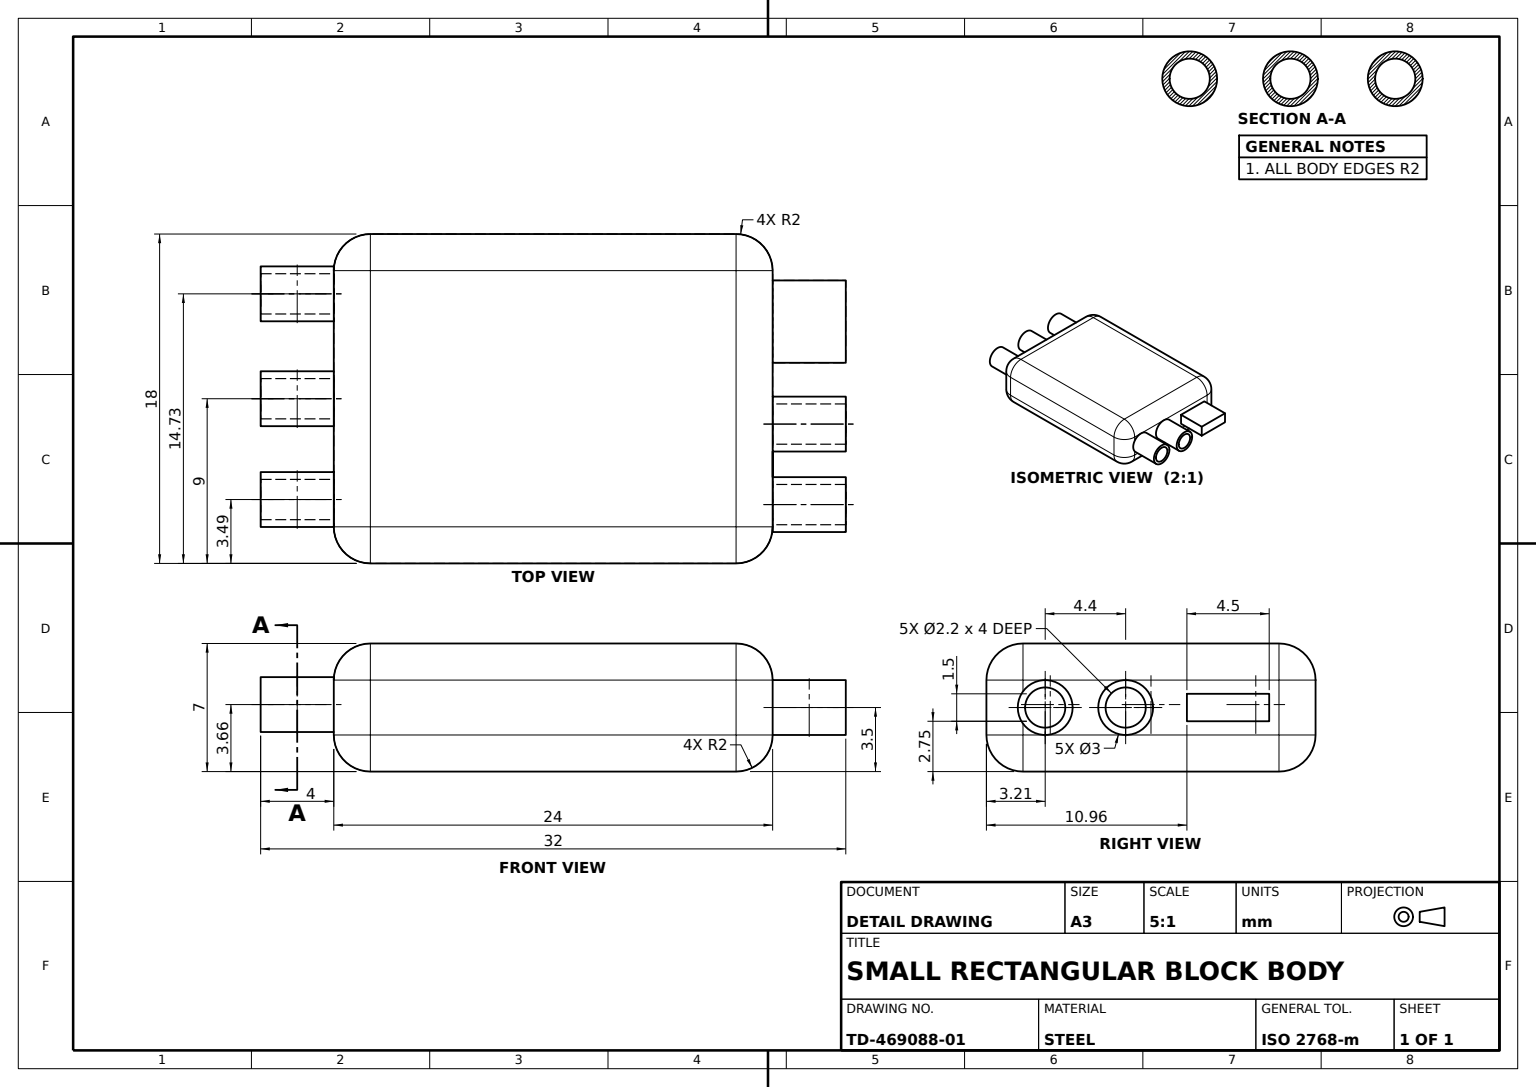
ISO-10303-21;
HEADER;
FILE_DESCRIPTION((''),'2;1');
FILE_NAME('','',(''),(''),'','','');
FILE_SCHEMA(('AUTOMOTIVE_DESIGN'));
ENDSEC;
DATA;
#1=APPLICATION_CONTEXT('');
#2=PRODUCT_CONTEXT('',#1,'mechanical');
#3=PRODUCT('','','',(#2));
#4=PRODUCT_DEFINITION_FORMATION('','',#3);
#5=PRODUCT_DEFINITION_CONTEXT('',#1,'design');
#6=PRODUCT_DEFINITION('','',#4,#5);
#7=PRODUCT_DEFINITION_SHAPE('','',#6);
#8=(LENGTH_UNIT()NAMED_UNIT(*)SI_UNIT(.MILLI.,.METRE.));
#9=(NAMED_UNIT(*)PLANE_ANGLE_UNIT()SI_UNIT($,.RADIAN.));
#10=(NAMED_UNIT(*)SI_UNIT($,.STERADIAN.)SOLID_ANGLE_UNIT());
#11=UNCERTAINTY_MEASURE_WITH_UNIT(LENGTH_MEASURE(1.E-05),#8,'distance_accuracy_value','');
#12=(GEOMETRIC_REPRESENTATION_CONTEXT(3)GLOBAL_UNCERTAINTY_ASSIGNED_CONTEXT((#11))GLOBAL_UNIT_ASSIGNED_CONTEXT((#8,#9,#10))REPRESENTATION_CONTEXT('',''));
#13=CARTESIAN_POINT('',(12.,2.,7.));
#14=VERTEX_POINT('',#13);
#15=CARTESIAN_POINT('',(12.,2.,5.785269));
#16=VERTEX_POINT('',#15);
#17=CARTESIAN_POINT('',(12.,2.,-7.));
#18=DIRECTION('',(0.,0.,-1.));
#19=VECTOR('',#18,1000.);
#20=LINE('',#17,#19);
#21=EDGE_CURVE('',#14,#16,#20,.T.);
#22=ORIENTED_EDGE('',*,*,#21,.T.);
#23=CARTESIAN_POINT('',(12.,2.619984,7.));
#24=VERTEX_POINT('',#23);
#25=CARTESIAN_POINT('',(12.,3.5,5.785269));
#26=DIRECTION('',(1.,0.,0.));
#27=AXIS2_PLACEMENT_3D('',#25,#26,#18);
#28=CIRCLE('',#27,1.5);
#29=EDGE_CURVE('',#24,#16,#28,.T.);
#30=ORIENTED_EDGE('',*,*,#29,.F.);
#31=CARTESIAN_POINT('',(12.,7.,7.));
#32=DIRECTION('',(0.,-1.,0.));
#33=VECTOR('',#32,1000.);
#34=LINE('',#31,#33);
#35=EDGE_CURVE('',#24,#14,#34,.T.);
#36=ORIENTED_EDGE('',*,*,#35,.T.);
#37=EDGE_LOOP('',(#22,#30,#36));
#38=FACE_OUTER_BOUND('',#37,.T.);
#39=CARTESIAN_POINT('',(12.,7.,-7.));
#40=DIRECTION('',(-1.,0.,0.));
#41=DIRECTION('',(0.,0.,1.));
#42=AXIS2_PLACEMENT_3D('',#39,#40,#41);
#43=PLANE('',#42);
#44=ADVANCED_FACE('',(#38),#43,.F.);
#45=CARTESIAN_POINT('',(12.,5.,7.));
#46=VERTEX_POINT('',#45);
#47=CARTESIAN_POINT('',(12.,4.380016,7.));
#48=VERTEX_POINT('',#47);
#49=EDGE_CURVE('',#46,#48,#34,.T.);
#50=ORIENTED_EDGE('',*,*,#49,.F.);
#51=CARTESIAN_POINT('',(10.,5.,9.));
#52=VERTEX_POINT('',#51);
#53=CARTESIAN_POINT('',(10.,5.,7.));
#54=AXIS2_PLACEMENT_3D('',#53,#32,#18);
#55=CIRCLE('',#54,2.);
#56=EDGE_CURVE('',#46,#52,#55,.T.);
#57=ORIENTED_EDGE('',*,*,#56,.T.);
#58=CARTESIAN_POINT('',(10.,2.,9.));
#59=VERTEX_POINT('',#58);
#60=CARTESIAN_POINT('',(10.,7.,9.));
#61=LINE('',#60,#33);
#62=EDGE_CURVE('',#52,#59,#61,.T.);
#63=ORIENTED_EDGE('',*,*,#62,.T.);
#64=CARTESIAN_POINT('',(10.,2.,7.));
#65=DIRECTION('',(0.,1.,0.));
#66=AXIS2_PLACEMENT_3D('',#64,#65,#18);
#67=CIRCLE('',#66,2.);
#68=EDGE_CURVE('',#59,#14,#67,.T.);
#69=ORIENTED_EDGE('',*,*,#68,.T.);
#70=ORIENTED_EDGE('',*,*,#35,.F.);
#71=EDGE_CURVE('',#48,#24,#34,.T.);
#72=ORIENTED_EDGE('',*,*,#71,.F.);
#73=EDGE_LOOP('',(#50,#57,#63,#69,#70,#72));
#74=FACE_OUTER_BOUND('',#73,.T.);
#75=CARTESIAN_POINT('',(10.,7.,7.));
#76=AXIS2_PLACEMENT_3D('',#75,#32,#18);
#77=CYLINDRICAL_SURFACE('',#76,2.);
#78=ADVANCED_FACE('',(#74),#77,.T.);
#79=CARTESIAN_POINT('',(-10.,0.,7.));
#80=VERTEX_POINT('',#79);
#81=CARTESIAN_POINT('',(-10.,0.,-7.));
#82=VERTEX_POINT('',#81);
#83=LINE('',#81,#19);
#84=EDGE_CURVE('',#80,#82,#83,.T.);
#85=ORIENTED_EDGE('',*,*,#84,.T.);
#86=CARTESIAN_POINT('',(10.,0.,-7.));
#87=VERTEX_POINT('',#86);
#88=VECTOR('',#26,1000.);
#89=LINE('',#86,#88);
#90=EDGE_CURVE('',#82,#87,#89,.T.);
#91=ORIENTED_EDGE('',*,*,#90,.T.);
#92=CARTESIAN_POINT('',(10.,0.,7.));
#93=VERTEX_POINT('',#92);
#94=VECTOR('',#41,1000.);
#95=LINE('',#92,#94);
#96=EDGE_CURVE('',#87,#93,#95,.T.);
#97=ORIENTED_EDGE('',*,*,#96,.T.);
#98=VECTOR('',#40,1000.);
#99=LINE('',#79,#98);
#100=EDGE_CURVE('',#93,#80,#99,.T.);
#101=ORIENTED_EDGE('',*,*,#100,.T.);
#102=EDGE_LOOP('',(#85,#91,#97,#101));
#103=FACE_OUTER_BOUND('',#102,.T.);
#104=AXIS2_PLACEMENT_3D('',#86,#32,#18);
#105=PLANE('',#104);
#106=ADVANCED_FACE('',(#103),#105,.T.);
#107=CARTESIAN_POINT('',(10.,7.,-7.));
#108=VERTEX_POINT('',#107);
#109=CARTESIAN_POINT('',(10.,5.,-9.));
#110=VERTEX_POINT('',#109);
#111=CARTESIAN_POINT('',(10.,5.,-7.));
#112=AXIS2_PLACEMENT_3D('',#111,#40,#41);
#113=CIRCLE('',#112,2.);
#114=EDGE_CURVE('',#108,#110,#113,.T.);
#115=ORIENTED_EDGE('',*,*,#114,.T.);
#116=CARTESIAN_POINT('',(-10.,5.,-9.));
#117=VERTEX_POINT('',#116);
#118=LINE('',#116,#88);
#119=EDGE_CURVE('',#117,#110,#118,.T.);
#120=ORIENTED_EDGE('',*,*,#119,.F.);
#121=CARTESIAN_POINT('',(-10.,7.,-7.));
#122=VERTEX_POINT('',#121);
#123=CARTESIAN_POINT('',(-10.,5.,-7.));
#124=AXIS2_PLACEMENT_3D('',#123,#40,#41);
#125=CIRCLE('',#124,2.);
#126=EDGE_CURVE('',#122,#117,#125,.T.);
#127=ORIENTED_EDGE('',*,*,#126,.F.);
#128=LINE('',#107,#98);
#129=EDGE_CURVE('',#108,#122,#128,.T.);
#130=ORIENTED_EDGE('',*,*,#129,.F.);
#131=EDGE_LOOP('',(#115,#120,#127,#130));
#132=FACE_OUTER_BOUND('',#131,.T.);
#133=CYLINDRICAL_SURFACE('',#112,2.);
#134=ADVANCED_FACE('',(#132),#133,.T.);
#135=CARTESIAN_POINT('',(-12.,5.,-5.053645));
#136=VERTEX_POINT('',#135);
#137=CARTESIAN_POINT('',(-12.,5.,-6.408669));
#138=VERTEX_POINT('',#137);
#139=CARTESIAN_POINT('',(-12.,3.661726,-5.731157));
#140=AXIS2_PLACEMENT_3D('',#139,#40,#41);
#141=CIRCLE('',#140,1.5);
#142=EDGE_CURVE('',#136,#138,#141,.T.);
#143=ORIENTED_EDGE('',*,*,#142,.F.);
#144=CARTESIAN_POINT('',(-12.,5.,-7.));
#145=LINE('',#144,#19);
#146=EDGE_CURVE('',#136,#138,#145,.T.);
#147=ORIENTED_EDGE('',*,*,#146,.T.);
#148=EDGE_LOOP('',(#143,#147));
#149=FACE_OUTER_BOUND('',#148,.T.);
#150=PLANE('',#140);
#151=ADVANCED_FACE('',(#149),#150,.F.);
#152=CARTESIAN_POINT('',(16.,4.25,-1.964278));
#153=VERTEX_POINT('',#152);
#154=CARTESIAN_POINT('',(12.,4.25,-1.964278));
#155=VERTEX_POINT('',#154);
#156=LINE('',#152,#98);
#157=EDGE_CURVE('',#153,#155,#156,.T.);
#158=ORIENTED_EDGE('',*,*,#157,.F.);
#159=CARTESIAN_POINT('',(16.,4.25,-6.464278));
#160=VERTEX_POINT('',#159);
#161=LINE('',#152,#94);
#162=EDGE_CURVE('',#160,#153,#161,.T.);
#163=ORIENTED_EDGE('',*,*,#162,.F.);
#164=CARTESIAN_POINT('',(12.,4.25,-6.464278));
#165=VERTEX_POINT('',#164);
#166=LINE('',#159,#98);
#167=EDGE_CURVE('',#160,#165,#166,.T.);
#168=ORIENTED_EDGE('',*,*,#167,.T.);
#169=LINE('',#154,#94);
#170=EDGE_CURVE('',#165,#155,#169,.T.);
#171=ORIENTED_EDGE('',*,*,#170,.T.);
#172=EDGE_LOOP('',(#158,#163,#168,#171));
#173=FACE_OUTER_BOUND('',#172,.T.);
#174=AXIS2_PLACEMENT_3D('',#152,#32,#18);
#175=PLANE('',#174);
#176=ADVANCED_FACE('',(#173),#175,.F.);
#177=VERTEX_POINT('',#144);
#178=AXIS2_PLACEMENT_3D('',#123,#41,#26);
#179=CIRCLE('',#178,2.);
#180=EDGE_CURVE('',#122,#177,#179,.T.);
#181=ORIENTED_EDGE('',*,*,#180,.F.);
#182=ORIENTED_EDGE('',*,*,#126,.T.);
#183=AXIS2_PLACEMENT_3D('',#123,#32,#18);
#184=CIRCLE('',#183,2.);
#185=EDGE_CURVE('',#177,#117,#184,.T.);
#186=ORIENTED_EDGE('',*,*,#185,.F.);
#187=EDGE_LOOP('',(#181,#182,#186));
#188=FACE_OUTER_BOUND('',#187,.T.);
#189=AXIS2_PLACEMENT_3D('',#123,#26,#18);
#190=SPHERICAL_SURFACE('',#189,2.);
#191=ADVANCED_FACE('',(#188),#190,.T.);
#192=CARTESIAN_POINT('',(-12.,4.461749,-7.));
#193=VERTEX_POINT('',#192);
#194=CARTESIAN_POINT('',(-12.,7.,-7.));
#195=LINE('',#194,#33);
#196=EDGE_CURVE('',#177,#193,#195,.T.);
#197=ORIENTED_EDGE('',*,*,#196,.F.);
#198=ORIENTED_EDGE('',*,*,#185,.T.);
#199=CARTESIAN_POINT('',(-10.,2.,-9.));
#200=VERTEX_POINT('',#199);
#201=CARTESIAN_POINT('',(-10.,7.,-9.));
#202=LINE('',#201,#33);
#203=EDGE_CURVE('',#117,#200,#202,.T.);
#204=ORIENTED_EDGE('',*,*,#203,.T.);
#205=CARTESIAN_POINT('',(-12.,2.,-7.));
#206=VERTEX_POINT('',#205);
#207=CARTESIAN_POINT('',(-10.,2.,-7.));
#208=AXIS2_PLACEMENT_3D('',#207,#65,#18);
#209=CIRCLE('',#208,2.);
#210=EDGE_CURVE('',#200,#206,#209,.T.);
#211=ORIENTED_EDGE('',*,*,#210,.T.);
#212=CARTESIAN_POINT('',(-12.,2.861703,-7.));
#213=VERTEX_POINT('',#212);
#214=EDGE_CURVE('',#213,#206,#195,.T.);
#215=ORIENTED_EDGE('',*,*,#214,.F.);
#216=EDGE_CURVE('',#193,#213,#195,.T.);
#217=ORIENTED_EDGE('',*,*,#216,.F.);
#218=EDGE_LOOP('',(#197,#198,#204,#211,#215,#217));
#219=FACE_OUTER_BOUND('',#218,.T.);
#220=AXIS2_PLACEMENT_3D('',#121,#32,#18);
#221=CYLINDRICAL_SURFACE('',#220,2.);
#222=ADVANCED_FACE('',(#219),#221,.T.);
#223=CARTESIAN_POINT('',(-10.,5.,9.));
#224=VERTEX_POINT('',#223);
#225=CARTESIAN_POINT('',(-12.,5.,7.));
#226=VERTEX_POINT('',#225);
#227=CARTESIAN_POINT('',(-10.,5.,7.));
#228=AXIS2_PLACEMENT_3D('',#227,#32,#18);
#229=CIRCLE('',#228,2.);
#230=EDGE_CURVE('',#224,#226,#229,.T.);
#231=ORIENTED_EDGE('',*,*,#230,.F.);
#232=CARTESIAN_POINT('',(-10.,7.,7.));
#233=VERTEX_POINT('',#232);
#234=AXIS2_PLACEMENT_3D('',#227,#40,#41);
#235=CIRCLE('',#234,2.);
#236=EDGE_CURVE('',#224,#233,#235,.T.);
#237=ORIENTED_EDGE('',*,*,#236,.T.);
#238=AXIS2_PLACEMENT_3D('',#227,#41,#26);
#239=CIRCLE('',#238,2.);
#240=EDGE_CURVE('',#233,#226,#239,.T.);
#241=ORIENTED_EDGE('',*,*,#240,.T.);
#242=EDGE_LOOP('',(#231,#237,#241));
#243=FACE_OUTER_BOUND('',#242,.T.);
#244=AXIS2_PLACEMENT_3D('',#227,#26,#18);
#245=SPHERICAL_SURFACE('',#244,2.);
#246=ADVANCED_FACE('',(#243),#245,.T.);
#247=CARTESIAN_POINT('',(16.,2.75,-6.464278));
#248=VERTEX_POINT('',#247);
#249=VECTOR('',#65,1000.);
#250=LINE('',#247,#249);
#251=EDGE_CURVE('',#248,#160,#250,.T.);
#252=ORIENTED_EDGE('',*,*,#251,.F.);
#253=CARTESIAN_POINT('',(12.,2.75,-6.464278));
#254=VERTEX_POINT('',#253);
#255=LINE('',#247,#98);
#256=EDGE_CURVE('',#248,#254,#255,.T.);
#257=ORIENTED_EDGE('',*,*,#256,.T.);
#258=LINE('',#253,#249);
#259=EDGE_CURVE('',#254,#165,#258,.T.);
#260=ORIENTED_EDGE('',*,*,#259,.T.);
#261=ORIENTED_EDGE('',*,*,#167,.F.);
#262=EDGE_LOOP('',(#252,#257,#260,#261));
#263=FACE_OUTER_BOUND('',#262,.T.);
#264=AXIS2_PLACEMENT_3D('',#247,#41,#26);
#265=PLANE('',#264);
#266=ADVANCED_FACE('',(#263),#265,.F.);
#267=CARTESIAN_POINT('',(10.,2.,-9.));
#268=VERTEX_POINT('',#267);
#269=CARTESIAN_POINT('',(10.,7.,-9.));
#270=LINE('',#269,#33);
#271=EDGE_CURVE('',#110,#268,#270,.T.);
#272=ORIENTED_EDGE('',*,*,#271,.F.);
#273=CARTESIAN_POINT('',(12.,5.,-7.));
#274=VERTEX_POINT('',#273);
#275=AXIS2_PLACEMENT_3D('',#111,#32,#18);
#276=CIRCLE('',#275,2.);
#277=EDGE_CURVE('',#110,#274,#276,.T.);
#278=ORIENTED_EDGE('',*,*,#277,.T.);
#279=VERTEX_POINT('',#17);
#280=LINE('',#39,#33);
#281=EDGE_CURVE('',#274,#279,#280,.T.);
#282=ORIENTED_EDGE('',*,*,#281,.T.);
#283=CARTESIAN_POINT('',(10.,2.,-7.));
#284=AXIS2_PLACEMENT_3D('',#283,#65,#18);
#285=CIRCLE('',#284,2.);
#286=EDGE_CURVE('',#279,#268,#285,.T.);
#287=ORIENTED_EDGE('',*,*,#286,.T.);
#288=EDGE_LOOP('',(#272,#278,#282,#287));
#289=FACE_OUTER_BOUND('',#288,.T.);
#290=AXIS2_PLACEMENT_3D('',#107,#32,#18);
#291=CYLINDRICAL_SURFACE('',#290,2.);
#292=ADVANCED_FACE('',(#289),#291,.T.);
#293=CARTESIAN_POINT('',(-12.,5.,0.677512));
#294=VERTEX_POINT('',#293);
#295=CARTESIAN_POINT('',(-12.,5.,-0.677512));
#296=VERTEX_POINT('',#295);
#297=CARTESIAN_POINT('',(-12.,3.661726,0.));
#298=AXIS2_PLACEMENT_3D('',#297,#40,#41);
#299=CIRCLE('',#298,1.5);
#300=EDGE_CURVE('',#294,#296,#299,.T.);
#301=ORIENTED_EDGE('',*,*,#300,.F.);
#302=EDGE_CURVE('',#294,#296,#145,.T.);
#303=ORIENTED_EDGE('',*,*,#302,.T.);
#304=EDGE_LOOP('',(#301,#303));
#305=FACE_OUTER_BOUND('',#304,.T.);
#306=PLANE('',#298);
#307=ADVANCED_FACE('',(#305),#306,.F.);
#308=CARTESIAN_POINT('',(-12.,3.661726,4.408784));
#309=VERTEX_POINT('',#308);
#310=CARTESIAN_POINT('',(-12.,3.661726,6.608784));
#311=VERTEX_POINT('',#310);
#312=CARTESIAN_POINT('',(-12.,3.661726,5.508784));
#313=AXIS2_PLACEMENT_3D('',#312,#40,#41);
#314=CIRCLE('',#313,1.1);
#315=EDGE_CURVE('',#309,#311,#314,.T.);
#316=ORIENTED_EDGE('',*,*,#315,.F.);
#317=CARTESIAN_POINT('',(-16.,3.661726,4.408784));
#318=VERTEX_POINT('',#317);
#319=LINE('',#317,#88);
#320=EDGE_CURVE('',#318,#309,#319,.T.);
#321=ORIENTED_EDGE('',*,*,#320,.F.);
#322=CARTESIAN_POINT('',(-16.,3.661726,6.608784));
#323=VERTEX_POINT('',#322);
#324=CARTESIAN_POINT('',(-16.,3.661726,5.508784));
#325=AXIS2_PLACEMENT_3D('',#324,#40,#41);
#326=CIRCLE('',#325,1.1);
#327=EDGE_CURVE('',#318,#323,#326,.T.);
#328=ORIENTED_EDGE('',*,*,#327,.T.);
#329=LINE('',#322,#88);
#330=EDGE_CURVE('',#323,#311,#329,.T.);
#331=ORIENTED_EDGE('',*,*,#330,.T.);
#332=EDGE_LOOP('',(#316,#321,#328,#331));
#333=FACE_OUTER_BOUND('',#332,.T.);
#334=AXIS2_PLACEMENT_3D('',#324,#26,#18);
#335=CYLINDRICAL_SURFACE('',#334,1.1);
#336=ADVANCED_FACE('',(#333),#335,.F.);
#337=VERTEX_POINT('',#75);
#338=AXIS2_PLACEMENT_3D('',#53,#41,#26);
#339=CIRCLE('',#338,2.);
#340=EDGE_CURVE('',#46,#337,#339,.T.);
#341=ORIENTED_EDGE('',*,*,#340,.T.);
#342=AXIS2_PLACEMENT_3D('',#53,#40,#41);
#343=CIRCLE('',#342,2.);
#344=EDGE_CURVE('',#52,#337,#343,.T.);
#345=ORIENTED_EDGE('',*,*,#344,.F.);
#346=ORIENTED_EDGE('',*,*,#56,.F.);
#347=EDGE_LOOP('',(#341,#345,#346));
#348=FACE_OUTER_BOUND('',#347,.T.);
#349=AXIS2_PLACEMENT_3D('',#53,#26,#18);
#350=SPHERICAL_SURFACE('',#349,2.);
#351=ADVANCED_FACE('',(#348),#350,.T.);
#352=CARTESIAN_POINT('',(16.,3.5,6.885269));
#353=VERTEX_POINT('',#352);
#354=CARTESIAN_POINT('',(12.,3.5,6.885269));
#355=VERTEX_POINT('',#354);
#356=LINE('',#352,#98);
#357=EDGE_CURVE('',#353,#355,#356,.T.);
#358=ORIENTED_EDGE('',*,*,#357,.F.);
#359=CARTESIAN_POINT('',(16.,3.5,4.685269));
#360=VERTEX_POINT('',#359);
#361=CARTESIAN_POINT('',(16.,3.5,5.785269));
#362=AXIS2_PLACEMENT_3D('',#361,#26,#18);
#363=CIRCLE('',#362,1.1);
#364=EDGE_CURVE('',#353,#360,#363,.T.);
#365=ORIENTED_EDGE('',*,*,#364,.T.);
#366=CARTESIAN_POINT('',(12.,3.5,4.685269));
#367=VERTEX_POINT('',#366);
#368=LINE('',#359,#98);
#369=EDGE_CURVE('',#360,#367,#368,.T.);
#370=ORIENTED_EDGE('',*,*,#369,.T.);
#371=CIRCLE('',#27,1.1);
#372=EDGE_CURVE('',#355,#367,#371,.T.);
#373=ORIENTED_EDGE('',*,*,#372,.F.);
#374=EDGE_LOOP('',(#358,#365,#370,#373));
#375=FACE_OUTER_BOUND('',#374,.T.);
#376=AXIS2_PLACEMENT_3D('',#361,#40,#41);
#377=CYLINDRICAL_SURFACE('',#376,1.1);
#378=ADVANCED_FACE('',(#375),#377,.F.);
#379=ORIENTED_EDGE('',*,*,#49,.T.);
#380=CARTESIAN_POINT('',(12.,5.,5.785269));
#381=VERTEX_POINT('',#380);
#382=EDGE_CURVE('',#381,#48,#28,.T.);
#383=ORIENTED_EDGE('',*,*,#382,.F.);
#384=LINE('',#273,#94);
#385=EDGE_CURVE('',#381,#46,#384,.T.);
#386=ORIENTED_EDGE('',*,*,#385,.T.);
#387=EDGE_LOOP('',(#379,#383,#386));
#388=FACE_OUTER_BOUND('',#387,.T.);
#389=ADVANCED_FACE('',(#388),#43,.F.);
#390=CARTESIAN_POINT('',(-16.,3.661726,-4.631157));
#391=VERTEX_POINT('',#390);
#392=CARTESIAN_POINT('',(-12.,3.661726,-4.631157));
#393=VERTEX_POINT('',#392);
#394=LINE('',#390,#88);
#395=EDGE_CURVE('',#391,#393,#394,.T.);
#396=ORIENTED_EDGE('',*,*,#395,.T.);
#397=CARTESIAN_POINT('',(-12.,3.661726,-6.831157));
#398=VERTEX_POINT('',#397);
#399=CIRCLE('',#140,1.1);
#400=EDGE_CURVE('',#398,#393,#399,.T.);
#401=ORIENTED_EDGE('',*,*,#400,.F.);
#402=CARTESIAN_POINT('',(-16.,3.661726,-6.831157));
#403=VERTEX_POINT('',#402);
#404=LINE('',#402,#88);
#405=EDGE_CURVE('',#403,#398,#404,.T.);
#406=ORIENTED_EDGE('',*,*,#405,.F.);
#407=CARTESIAN_POINT('',(-16.,3.661726,-5.731157));
#408=AXIS2_PLACEMENT_3D('',#407,#40,#41);
#409=CIRCLE('',#408,1.1);
#410=EDGE_CURVE('',#403,#391,#409,.T.);
#411=ORIENTED_EDGE('',*,*,#410,.T.);
#412=EDGE_LOOP('',(#396,#401,#406,#411));
#413=FACE_OUTER_BOUND('',#412,.T.);
#414=AXIS2_PLACEMENT_3D('',#407,#26,#18);
#415=CYLINDRICAL_SURFACE('',#414,1.1);
#416=ADVANCED_FACE('',(#413),#415,.F.);
#417=CARTESIAN_POINT('',(-12.,3.661726,-4.231157));
#418=VERTEX_POINT('',#417);
#419=EDGE_CURVE('',#213,#418,#141,.T.);
#420=ORIENTED_EDGE('',*,*,#419,.T.);
#421=CARTESIAN_POINT('',(-16.,3.661726,-4.231157));
#422=VERTEX_POINT('',#421);
#423=LINE('',#421,#88);
#424=EDGE_CURVE('',#422,#418,#423,.T.);
#425=ORIENTED_EDGE('',*,*,#424,.F.);
#426=CARTESIAN_POINT('',(-16.,3.661726,-7.231157));
#427=VERTEX_POINT('',#426);
#428=CIRCLE('',#408,1.5);
#429=EDGE_CURVE('',#427,#422,#428,.T.);
#430=ORIENTED_EDGE('',*,*,#429,.F.);
#431=CARTESIAN_POINT('',(-12.,3.661726,-7.231157));
#432=VERTEX_POINT('',#431);
#433=LINE('',#426,#88);
#434=EDGE_CURVE('',#427,#432,#433,.T.);
#435=ORIENTED_EDGE('',*,*,#434,.T.);
#436=EDGE_CURVE('',#432,#213,#141,.T.);
#437=ORIENTED_EDGE('',*,*,#436,.T.);
#438=EDGE_LOOP('',(#420,#425,#430,#435,#437));
#439=FACE_OUTER_BOUND('',#438,.T.);
#440=CYLINDRICAL_SURFACE('',#414,1.5);
#441=ADVANCED_FACE('',(#439),#440,.T.);
#442=CARTESIAN_POINT('',(16.,3.5,2.485269));
#443=VERTEX_POINT('',#442);
#444=CARTESIAN_POINT('',(16.,3.5,0.285269));
#445=VERTEX_POINT('',#444);
#446=CARTESIAN_POINT('',(16.,3.5,1.385269));
#447=AXIS2_PLACEMENT_3D('',#446,#26,#18);
#448=CIRCLE('',#447,1.1);
#449=EDGE_CURVE('',#443,#445,#448,.T.);
#450=ORIENTED_EDGE('',*,*,#449,.F.);
#451=EDGE_CURVE('',#445,#443,#448,.T.);
#452=ORIENTED_EDGE('',*,*,#451,.F.);
#453=EDGE_LOOP('',(#450,#452));
#454=FACE_BOUND('',#453,.T.);
#455=CARTESIAN_POINT('',(16.,3.5,-0.114731));
#456=VERTEX_POINT('',#455);
#457=CARTESIAN_POINT('',(16.,3.5,2.885269));
#458=VERTEX_POINT('',#457);
#459=CIRCLE('',#447,1.5);
#460=EDGE_CURVE('',#456,#458,#459,.T.);
#461=ORIENTED_EDGE('',*,*,#460,.T.);
#462=EDGE_CURVE('',#458,#456,#459,.T.);
#463=ORIENTED_EDGE('',*,*,#462,.T.);
#464=EDGE_LOOP('',(#461,#463));
#465=FACE_OUTER_BOUND('',#464,.T.);
#466=PLANE('',#447);
#467=ADVANCED_FACE('',(#454,#465),#466,.T.);
#468=CARTESIAN_POINT('',(-12.,3.499631,7.));
#469=VERTEX_POINT('',#468);
#470=CARTESIAN_POINT('',(-12.,2.,7.));
#471=VERTEX_POINT('',#470);
#472=CARTESIAN_POINT('',(-12.,7.,7.));
#473=LINE('',#472,#33);
#474=EDGE_CURVE('',#469,#471,#473,.T.);
#475=ORIENTED_EDGE('',*,*,#474,.T.);
#476=CARTESIAN_POINT('',(-10.,2.,9.));
#477=VERTEX_POINT('',#476);
#478=CARTESIAN_POINT('',(-10.,2.,7.));
#479=AXIS2_PLACEMENT_3D('',#478,#65,#18);
#480=CIRCLE('',#479,2.);
#481=EDGE_CURVE('',#471,#477,#480,.T.);
#482=ORIENTED_EDGE('',*,*,#481,.T.);
#483=CARTESIAN_POINT('',(-10.,7.,9.));
#484=LINE('',#483,#33);
#485=EDGE_CURVE('',#224,#477,#484,.T.);
#486=ORIENTED_EDGE('',*,*,#485,.F.);
#487=ORIENTED_EDGE('',*,*,#230,.T.);
#488=CARTESIAN_POINT('',(-12.,3.82382,7.));
#489=VERTEX_POINT('',#488);
#490=EDGE_CURVE('',#226,#489,#473,.T.);
#491=ORIENTED_EDGE('',*,*,#490,.T.);
#492=EDGE_CURVE('',#489,#469,#473,.T.);
#493=ORIENTED_EDGE('',*,*,#492,.T.);
#494=EDGE_LOOP('',(#475,#482,#486,#487,#491,#493));
#495=FACE_OUTER_BOUND('',#494,.T.);
#496=AXIS2_PLACEMENT_3D('',#232,#32,#18);
#497=CYLINDRICAL_SURFACE('',#496,2.);
#498=ADVANCED_FACE('',(#495),#497,.T.);
#499=ORIENTED_EDGE('',*,*,#210,.F.);
#500=AXIS2_PLACEMENT_3D('',#207,#40,#32);
#501=CIRCLE('',#500,2.);
#502=EDGE_CURVE('',#200,#82,#501,.T.);
#503=ORIENTED_EDGE('',*,*,#502,.T.);
#504=AXIS2_PLACEMENT_3D('',#207,#41,#26);
#505=CIRCLE('',#504,2.);
#506=EDGE_CURVE('',#206,#82,#505,.T.);
#507=ORIENTED_EDGE('',*,*,#506,.F.);
#508=EDGE_LOOP('',(#499,#503,#507));
#509=FACE_OUTER_BOUND('',#508,.T.);
#510=AXIS2_PLACEMENT_3D('',#207,#26,#18);
#511=SPHERICAL_SURFACE('',#510,2.);
#512=ADVANCED_FACE('',(#509),#511,.T.);
#513=LINE('',#470,#94);
#514=EDGE_CURVE('',#206,#471,#513,.T.);
#515=ORIENTED_EDGE('',*,*,#514,.F.);
#516=ORIENTED_EDGE('',*,*,#506,.T.);
#517=ORIENTED_EDGE('',*,*,#84,.F.);
#518=AXIS2_PLACEMENT_3D('',#478,#41,#32);
#519=CIRCLE('',#518,2.);
#520=EDGE_CURVE('',#471,#80,#519,.T.);
#521=ORIENTED_EDGE('',*,*,#520,.F.);
#522=EDGE_LOOP('',(#515,#516,#517,#521));
#523=FACE_OUTER_BOUND('',#522,.T.);
#524=AXIS2_PLACEMENT_3D('',#207,#18,#40);
#525=CYLINDRICAL_SURFACE('',#524,2.);
#526=ADVANCED_FACE('',(#523),#525,.T.);
#527=CARTESIAN_POINT('',(-16.,3.661726,1.5));
#528=VERTEX_POINT('',#527);
#529=CARTESIAN_POINT('',(-12.,3.661726,1.5));
#530=VERTEX_POINT('',#529);
#531=LINE('',#527,#88);
#532=EDGE_CURVE('',#528,#530,#531,.T.);
#533=ORIENTED_EDGE('',*,*,#532,.T.);
#534=EDGE_CURVE('',#530,#294,#299,.T.);
#535=ORIENTED_EDGE('',*,*,#534,.T.);
#536=ORIENTED_EDGE('',*,*,#300,.T.);
#537=CARTESIAN_POINT('',(-12.,3.661726,-1.5));
#538=VERTEX_POINT('',#537);
#539=EDGE_CURVE('',#296,#538,#299,.T.);
#540=ORIENTED_EDGE('',*,*,#539,.T.);
#541=CARTESIAN_POINT('',(-16.,3.661726,-1.5));
#542=VERTEX_POINT('',#541);
#543=LINE('',#541,#88);
#544=EDGE_CURVE('',#542,#538,#543,.T.);
#545=ORIENTED_EDGE('',*,*,#544,.F.);
#546=CARTESIAN_POINT('',(-16.,3.661726,0.));
#547=AXIS2_PLACEMENT_3D('',#546,#40,#41);
#548=CIRCLE('',#547,1.5);
#549=EDGE_CURVE('',#528,#542,#548,.T.);
#550=ORIENTED_EDGE('',*,*,#549,.F.);
#551=EDGE_LOOP('',(#533,#535,#536,#540,#545,#550));
#552=FACE_OUTER_BOUND('',#551,.T.);
#553=AXIS2_PLACEMENT_3D('',#546,#26,#18);
#554=CYLINDRICAL_SURFACE('',#553,1.5);
#555=ADVANCED_FACE('',(#552),#554,.T.);
#556=CARTESIAN_POINT('',(-16.,3.661726,1.1));
#557=VERTEX_POINT('',#556);
#558=CARTESIAN_POINT('',(-12.,3.661726,1.1));
#559=VERTEX_POINT('',#558);
#560=LINE('',#556,#88);
#561=EDGE_CURVE('',#557,#559,#560,.T.);
#562=ORIENTED_EDGE('',*,*,#561,.T.);
#563=CARTESIAN_POINT('',(-12.,3.661726,-1.1));
#564=VERTEX_POINT('',#563);
#565=CIRCLE('',#298,1.1);
#566=EDGE_CURVE('',#564,#559,#565,.T.);
#567=ORIENTED_EDGE('',*,*,#566,.F.);
#568=CARTESIAN_POINT('',(-16.,3.661726,-1.1));
#569=VERTEX_POINT('',#568);
#570=LINE('',#568,#88);
#571=EDGE_CURVE('',#569,#564,#570,.T.);
#572=ORIENTED_EDGE('',*,*,#571,.F.);
#573=CIRCLE('',#547,1.1);
#574=EDGE_CURVE('',#569,#557,#573,.T.);
#575=ORIENTED_EDGE('',*,*,#574,.T.);
#576=EDGE_LOOP('',(#562,#567,#572,#575));
#577=FACE_OUTER_BOUND('',#576,.T.);
#578=CYLINDRICAL_SURFACE('',#553,1.1);
#579=ADVANCED_FACE('',(#577),#578,.F.);
#580=CARTESIAN_POINT('',(-16.,3.661726,7.008784));
#581=VERTEX_POINT('',#580);
#582=CARTESIAN_POINT('',(-12.,3.661726,7.008784));
#583=VERTEX_POINT('',#582);
#584=LINE('',#580,#88);
#585=EDGE_CURVE('',#581,#583,#584,.T.);
#586=ORIENTED_EDGE('',*,*,#585,.F.);
#587=CARTESIAN_POINT('',(-16.,3.661726,4.008784));
#588=VERTEX_POINT('',#587);
#589=CIRCLE('',#325,1.5);
#590=EDGE_CURVE('',#588,#581,#589,.T.);
#591=ORIENTED_EDGE('',*,*,#590,.F.);
#592=CARTESIAN_POINT('',(-12.,3.661726,4.008784));
#593=VERTEX_POINT('',#592);
#594=LINE('',#587,#88);
#595=EDGE_CURVE('',#588,#593,#594,.T.);
#596=ORIENTED_EDGE('',*,*,#595,.T.);
#597=CIRCLE('',#313,1.5);
#598=EDGE_CURVE('',#593,#469,#597,.T.);
#599=ORIENTED_EDGE('',*,*,#598,.T.);
#600=EDGE_CURVE('',#469,#583,#597,.T.);
#601=ORIENTED_EDGE('',*,*,#600,.T.);
#602=EDGE_LOOP('',(#586,#591,#596,#599,#601));
#603=FACE_OUTER_BOUND('',#602,.T.);
#604=CYLINDRICAL_SURFACE('',#334,1.5);
#605=ADVANCED_FACE('',(#603),#604,.T.);
#606=EDGE_CURVE('',#311,#309,#314,.T.);
#607=ORIENTED_EDGE('',*,*,#606,.T.);
#608=ORIENTED_EDGE('',*,*,#315,.T.);
#609=EDGE_LOOP('',(#607,#608));
#610=FACE_OUTER_BOUND('',#609,.T.);
#611=AXIS2_PLACEMENT_3D('',#194,#26,#18);
#612=PLANE('',#611);
#613=ADVANCED_FACE('',(#610),#612,.F.);
#614=CARTESIAN_POINT('',(12.,5.,1.385269));
#615=VERTEX_POINT('',#614);
#616=CARTESIAN_POINT('',(12.,3.5,2.885269));
#617=VERTEX_POINT('',#616);
#618=CARTESIAN_POINT('',(12.,3.5,1.385269));
#619=AXIS2_PLACEMENT_3D('',#618,#26,#18);
#620=CIRCLE('',#619,1.5);
#621=EDGE_CURVE('',#615,#617,#620,.T.);
#622=ORIENTED_EDGE('',*,*,#621,.F.);
#623=EDGE_CURVE('',#615,#381,#384,.T.);
#624=ORIENTED_EDGE('',*,*,#623,.T.);
#625=CARTESIAN_POINT('',(12.,3.5,4.285269));
#626=VERTEX_POINT('',#625);
#627=EDGE_CURVE('',#626,#381,#28,.T.);
#628=ORIENTED_EDGE('',*,*,#627,.F.);
#629=EDGE_CURVE('',#16,#626,#28,.T.);
#630=ORIENTED_EDGE('',*,*,#629,.F.);
#631=CARTESIAN_POINT('',(12.,2.,1.385269));
#632=VERTEX_POINT('',#631);
#633=EDGE_CURVE('',#16,#632,#20,.T.);
#634=ORIENTED_EDGE('',*,*,#633,.T.);
#635=EDGE_CURVE('',#617,#632,#620,.T.);
#636=ORIENTED_EDGE('',*,*,#635,.F.);
#637=EDGE_LOOP('',(#622,#624,#628,#630,#634,#636));
#638=FACE_OUTER_BOUND('',#637,.T.);
#639=ADVANCED_FACE('',(#638),#43,.F.);
#640=CARTESIAN_POINT('',(16.,2.75,-1.964278));
#641=VERTEX_POINT('',#640);
#642=LINE('',#640,#19);
#643=EDGE_CURVE('',#641,#248,#642,.T.);
#644=ORIENTED_EDGE('',*,*,#643,.T.);
#645=ORIENTED_EDGE('',*,*,#251,.T.);
#646=ORIENTED_EDGE('',*,*,#162,.T.);
#647=LINE('',#640,#33);
#648=EDGE_CURVE('',#153,#641,#647,.T.);
#649=ORIENTED_EDGE('',*,*,#648,.T.);
#650=EDGE_LOOP('',(#644,#645,#646,#649));
#651=FACE_OUTER_BOUND('',#650,.T.);
#652=CARTESIAN_POINT('',(16.,0.,0.));
#653=AXIS2_PLACEMENT_3D('',#652,#40,#41);
#654=PLANE('',#653);
#655=ADVANCED_FACE('',(#651),#654,.F.);
#656=ORIENTED_EDGE('',*,*,#180,.T.);
#657=EDGE_CURVE('',#138,#177,#145,.T.);
#658=ORIENTED_EDGE('',*,*,#657,.F.);
#659=ORIENTED_EDGE('',*,*,#146,.F.);
#660=EDGE_CURVE('',#296,#136,#145,.T.);
#661=ORIENTED_EDGE('',*,*,#660,.F.);
#662=ORIENTED_EDGE('',*,*,#302,.F.);
#663=CARTESIAN_POINT('',(-12.,5.,4.831272));
#664=VERTEX_POINT('',#663);
#665=EDGE_CURVE('',#664,#294,#145,.T.);
#666=ORIENTED_EDGE('',*,*,#665,.F.);
#667=CARTESIAN_POINT('',(-12.,5.,6.186296));
#668=VERTEX_POINT('',#667);
#669=EDGE_CURVE('',#668,#664,#145,.T.);
#670=ORIENTED_EDGE('',*,*,#669,.F.);
#671=EDGE_CURVE('',#226,#668,#145,.T.);
#672=ORIENTED_EDGE('',*,*,#671,.F.);
#673=ORIENTED_EDGE('',*,*,#240,.F.);
#674=LINE('',#121,#94);
#675=EDGE_CURVE('',#122,#233,#674,.T.);
#676=ORIENTED_EDGE('',*,*,#675,.F.);
#677=EDGE_LOOP('',(#656,#658,#659,#661,#662,#666,#670,#672,#673,#676));
#678=FACE_OUTER_BOUND('',#677,.T.);
#679=CYLINDRICAL_SURFACE('',#178,2.);
#680=ADVANCED_FACE('',(#678),#679,.T.);
#681=LINE('',#457,#98);
#682=EDGE_CURVE('',#458,#617,#681,.T.);
#683=ORIENTED_EDGE('',*,*,#682,.F.);
#684=ORIENTED_EDGE('',*,*,#460,.F.);
#685=CARTESIAN_POINT('',(12.,3.5,-0.114731));
#686=VERTEX_POINT('',#685);
#687=LINE('',#455,#98);
#688=EDGE_CURVE('',#456,#686,#687,.T.);
#689=ORIENTED_EDGE('',*,*,#688,.T.);
#690=EDGE_CURVE('',#686,#615,#620,.T.);
#691=ORIENTED_EDGE('',*,*,#690,.T.);
#692=ORIENTED_EDGE('',*,*,#621,.T.);
#693=EDGE_LOOP('',(#683,#684,#689,#691,#692));
#694=FACE_OUTER_BOUND('',#693,.T.);
#695=AXIS2_PLACEMENT_3D('',#446,#40,#41);
#696=CYLINDRICAL_SURFACE('',#695,1.5);
#697=ADVANCED_FACE('',(#694),#696,.T.);
#698=ORIENTED_EDGE('',*,*,#100,.F.);
#699=AXIS2_PLACEMENT_3D('',#64,#40,#41);
#700=CIRCLE('',#699,2.);
#701=EDGE_CURVE('',#93,#59,#700,.T.);
#702=ORIENTED_EDGE('',*,*,#701,.T.);
#703=LINE('',#58,#88);
#704=EDGE_CURVE('',#477,#59,#703,.T.);
#705=ORIENTED_EDGE('',*,*,#704,.F.);
#706=AXIS2_PLACEMENT_3D('',#478,#40,#41);
#707=CIRCLE('',#706,2.);
#708=EDGE_CURVE('',#80,#477,#707,.T.);
#709=ORIENTED_EDGE('',*,*,#708,.F.);
#710=EDGE_LOOP('',(#698,#702,#705,#709));
#711=FACE_OUTER_BOUND('',#710,.T.);
#712=CYLINDRICAL_SURFACE('',#706,2.);
#713=ADVANCED_FACE('',(#711),#712,.T.);
#714=ORIENTED_EDGE('',*,*,#157,.T.);
#715=CARTESIAN_POINT('',(12.,2.75,-1.964278));
#716=VERTEX_POINT('',#715);
#717=LINE('',#715,#33);
#718=EDGE_CURVE('',#155,#716,#717,.T.);
#719=ORIENTED_EDGE('',*,*,#718,.T.);
#720=LINE('',#640,#98);
#721=EDGE_CURVE('',#641,#716,#720,.T.);
#722=ORIENTED_EDGE('',*,*,#721,.F.);
#723=ORIENTED_EDGE('',*,*,#648,.F.);
#724=EDGE_LOOP('',(#714,#719,#722,#723));
#725=FACE_OUTER_BOUND('',#724,.T.);
#726=AXIS2_PLACEMENT_3D('',#640,#18,#40);
#727=PLANE('',#726);
#728=ADVANCED_FACE('',(#725),#727,.F.);
#729=ORIENTED_EDGE('',*,*,#492,.F.);
#730=EDGE_CURVE('',#583,#489,#597,.T.);
#731=ORIENTED_EDGE('',*,*,#730,.F.);
#732=ORIENTED_EDGE('',*,*,#600,.F.);
#733=EDGE_LOOP('',(#729,#731,#732));
#734=FACE_OUTER_BOUND('',#733,.T.);
#735=PLANE('',#313);
#736=ADVANCED_FACE('',(#734),#735,.F.);
#737=ORIENTED_EDGE('',*,*,#364,.F.);
#738=EDGE_CURVE('',#360,#353,#363,.T.);
#739=ORIENTED_EDGE('',*,*,#738,.F.);
#740=EDGE_LOOP('',(#737,#739));
#741=FACE_BOUND('',#740,.T.);
#742=CARTESIAN_POINT('',(16.,3.5,4.285269));
#743=VERTEX_POINT('',#742);
#744=CARTESIAN_POINT('',(16.,3.5,7.285269));
#745=VERTEX_POINT('',#744);
#746=CIRCLE('',#362,1.5);
#747=EDGE_CURVE('',#743,#745,#746,.T.);
#748=ORIENTED_EDGE('',*,*,#747,.T.);
#749=EDGE_CURVE('',#745,#743,#746,.T.);
#750=ORIENTED_EDGE('',*,*,#749,.T.);
#751=EDGE_LOOP('',(#748,#750));
#752=FACE_OUTER_BOUND('',#751,.T.);
#753=PLANE('',#362);
#754=ADVANCED_FACE('',(#741,#752),#753,.T.);
#755=CARTESIAN_POINT('',(12.,3.5,0.285269));
#756=VERTEX_POINT('',#755);
#757=LINE('',#444,#98);
#758=EDGE_CURVE('',#445,#756,#757,.T.);
#759=ORIENTED_EDGE('',*,*,#758,.F.);
#760=ORIENTED_EDGE('',*,*,#451,.T.);
#761=CARTESIAN_POINT('',(12.,3.5,2.485269));
#762=VERTEX_POINT('',#761);
#763=LINE('',#442,#98);
#764=EDGE_CURVE('',#443,#762,#763,.T.);
#765=ORIENTED_EDGE('',*,*,#764,.T.);
#766=CIRCLE('',#619,1.1);
#767=EDGE_CURVE('',#756,#762,#766,.T.);
#768=ORIENTED_EDGE('',*,*,#767,.F.);
#769=EDGE_LOOP('',(#759,#760,#765,#768));
#770=FACE_OUTER_BOUND('',#769,.T.);
#771=CYLINDRICAL_SURFACE('',#695,1.1);
#772=ADVANCED_FACE('',(#770),#771,.F.);
#773=ORIENTED_EDGE('',*,*,#544,.T.);
#774=EDGE_CURVE('',#538,#530,#299,.T.);
#775=ORIENTED_EDGE('',*,*,#774,.T.);
#776=ORIENTED_EDGE('',*,*,#532,.F.);
#777=EDGE_CURVE('',#542,#528,#548,.T.);
#778=ORIENTED_EDGE('',*,*,#777,.F.);
#779=EDGE_LOOP('',(#773,#775,#776,#778));
#780=FACE_OUTER_BOUND('',#779,.T.);
#781=ADVANCED_FACE('',(#780),#554,.T.);
#782=ORIENTED_EDGE('',*,*,#520,.T.);
#783=ORIENTED_EDGE('',*,*,#708,.T.);
#784=ORIENTED_EDGE('',*,*,#481,.F.);
#785=EDGE_LOOP('',(#782,#783,#784));
#786=FACE_OUTER_BOUND('',#785,.T.);
#787=AXIS2_PLACEMENT_3D('',#478,#26,#18);
#788=SPHERICAL_SURFACE('',#787,2.);
#789=ADVANCED_FACE('',(#786),#788,.T.);
#790=ORIENTED_EDGE('',*,*,#566,.T.);
#791=EDGE_CURVE('',#559,#564,#565,.T.);
#792=ORIENTED_EDGE('',*,*,#791,.T.);
#793=EDGE_LOOP('',(#790,#792));
#794=FACE_OUTER_BOUND('',#793,.T.);
#795=ADVANCED_FACE('',(#794),#612,.F.);
#796=EDGE_CURVE('',#193,#432,#141,.T.);
#797=ORIENTED_EDGE('',*,*,#796,.T.);
#798=ORIENTED_EDGE('',*,*,#434,.F.);
#799=EDGE_CURVE('',#422,#427,#428,.T.);
#800=ORIENTED_EDGE('',*,*,#799,.F.);
#801=ORIENTED_EDGE('',*,*,#424,.T.);
#802=EDGE_CURVE('',#418,#136,#141,.T.);
#803=ORIENTED_EDGE('',*,*,#802,.T.);
#804=ORIENTED_EDGE('',*,*,#142,.T.);
#805=EDGE_CURVE('',#138,#193,#141,.T.);
#806=ORIENTED_EDGE('',*,*,#805,.T.);
#807=EDGE_LOOP('',(#797,#798,#800,#801,#803,#804,#806));
#808=FACE_OUTER_BOUND('',#807,.T.);
#809=ADVANCED_FACE('',(#808),#440,.T.);
#810=ORIENTED_EDGE('',*,*,#585,.T.);
#811=ORIENTED_EDGE('',*,*,#730,.T.);
#812=EDGE_CURVE('',#489,#668,#597,.T.);
#813=ORIENTED_EDGE('',*,*,#812,.T.);
#814=EDGE_CURVE('',#668,#664,#597,.T.);
#815=ORIENTED_EDGE('',*,*,#814,.T.);
#816=EDGE_CURVE('',#664,#593,#597,.T.);
#817=ORIENTED_EDGE('',*,*,#816,.T.);
#818=ORIENTED_EDGE('',*,*,#595,.F.);
#819=EDGE_CURVE('',#581,#588,#589,.T.);
#820=ORIENTED_EDGE('',*,*,#819,.F.);
#821=EDGE_LOOP('',(#810,#811,#813,#815,#817,#818,#820));
#822=FACE_OUTER_BOUND('',#821,.T.);
#823=ADVANCED_FACE('',(#822),#604,.T.);
#824=ORIENTED_EDGE('',*,*,#129,.T.);
#825=ORIENTED_EDGE('',*,*,#675,.T.);
#826=LINE('',#75,#88);
#827=EDGE_CURVE('',#233,#337,#826,.T.);
#828=ORIENTED_EDGE('',*,*,#827,.T.);
#829=LINE('',#107,#19);
#830=EDGE_CURVE('',#337,#108,#829,.T.);
#831=ORIENTED_EDGE('',*,*,#830,.T.);
#832=EDGE_LOOP('',(#824,#825,#828,#831));
#833=FACE_OUTER_BOUND('',#832,.T.);
#834=PLANE('',#290);
#835=ADVANCED_FACE('',(#833),#834,.F.);
#836=ORIENTED_EDGE('',*,*,#170,.F.);
#837=ORIENTED_EDGE('',*,*,#259,.F.);
#838=LINE('',#715,#19);
#839=EDGE_CURVE('',#716,#254,#838,.T.);
#840=ORIENTED_EDGE('',*,*,#839,.F.);
#841=ORIENTED_EDGE('',*,*,#718,.F.);
#842=EDGE_LOOP('',(#836,#837,#840,#841));
#843=FACE_BOUND('',#842,.T.);
#844=ORIENTED_EDGE('',*,*,#690,.F.);
#845=EDGE_CURVE('',#632,#686,#620,.T.);
#846=ORIENTED_EDGE('',*,*,#845,.F.);
#847=EDGE_CURVE('',#632,#279,#20,.T.);
#848=ORIENTED_EDGE('',*,*,#847,.T.);
#849=ORIENTED_EDGE('',*,*,#281,.F.);
#850=EDGE_CURVE('',#274,#615,#384,.T.);
#851=ORIENTED_EDGE('',*,*,#850,.T.);
#852=EDGE_LOOP('',(#844,#846,#848,#849,#851));
#853=FACE_OUTER_BOUND('',#852,.T.);
#854=ADVANCED_FACE('',(#843,#853),#43,.F.);
#855=ORIENTED_EDGE('',*,*,#344,.T.);
#856=ORIENTED_EDGE('',*,*,#827,.F.);
#857=ORIENTED_EDGE('',*,*,#236,.F.);
#858=LINE('',#223,#98);
#859=EDGE_CURVE('',#52,#224,#858,.T.);
#860=ORIENTED_EDGE('',*,*,#859,.F.);
#861=EDGE_LOOP('',(#855,#856,#857,#860));
#862=FACE_OUTER_BOUND('',#861,.T.);
#863=CYLINDRICAL_SURFACE('',#349,2.);
#864=ADVANCED_FACE('',(#862),#863,.T.);
#865=ORIENTED_EDGE('',*,*,#277,.F.);
#866=ORIENTED_EDGE('',*,*,#114,.F.);
#867=AXIS2_PLACEMENT_3D('',#111,#41,#26);
#868=CIRCLE('',#867,2.);
#869=EDGE_CURVE('',#274,#108,#868,.T.);
#870=ORIENTED_EDGE('',*,*,#869,.F.);
#871=EDGE_LOOP('',(#865,#866,#870));
#872=FACE_OUTER_BOUND('',#871,.T.);
#873=AXIS2_PLACEMENT_3D('',#111,#26,#18);
#874=SPHERICAL_SURFACE('',#873,2.);
#875=ADVANCED_FACE('',(#872),#874,.T.);
#876=ORIENTED_EDGE('',*,*,#796,.F.);
#877=ORIENTED_EDGE('',*,*,#216,.T.);
#878=ORIENTED_EDGE('',*,*,#436,.F.);
#879=EDGE_LOOP('',(#876,#877,#878));
#880=FACE_OUTER_BOUND('',#879,.T.);
#881=ADVANCED_FACE('',(#880),#150,.F.);
#882=ORIENTED_EDGE('',*,*,#669,.T.);
#883=ORIENTED_EDGE('',*,*,#814,.F.);
#884=EDGE_LOOP('',(#882,#883));
#885=FACE_OUTER_BOUND('',#884,.T.);
#886=ADVANCED_FACE('',(#885),#735,.F.);
#887=ORIENTED_EDGE('',*,*,#657,.T.);
#888=ORIENTED_EDGE('',*,*,#196,.T.);
#889=ORIENTED_EDGE('',*,*,#805,.F.);
#890=EDGE_LOOP('',(#887,#888,#889));
#891=FACE_OUTER_BOUND('',#890,.T.);
#892=ADVANCED_FACE('',(#891),#612,.F.);
#893=CARTESIAN_POINT('',(12.,3.5,7.285269));
#894=VERTEX_POINT('',#893);
#895=EDGE_CURVE('',#894,#24,#28,.T.);
#896=ORIENTED_EDGE('',*,*,#895,.F.);
#897=EDGE_CURVE('',#48,#894,#28,.T.);
#898=ORIENTED_EDGE('',*,*,#897,.F.);
#899=ORIENTED_EDGE('',*,*,#71,.T.);
#900=EDGE_LOOP('',(#896,#898,#899));
#901=FACE_OUTER_BOUND('',#900,.T.);
#902=PLANE('',#27);
#903=ADVANCED_FACE('',(#901),#902,.F.);
#904=AXIS2_PLACEMENT_3D('',#283,#41,#26);
#905=CIRCLE('',#904,2.);
#906=EDGE_CURVE('',#87,#279,#905,.T.);
#907=ORIENTED_EDGE('',*,*,#906,.F.);
#908=AXIS2_PLACEMENT_3D('',#283,#40,#41);
#909=CIRCLE('',#908,2.);
#910=EDGE_CURVE('',#268,#87,#909,.T.);
#911=ORIENTED_EDGE('',*,*,#910,.F.);
#912=ORIENTED_EDGE('',*,*,#286,.F.);
#913=EDGE_LOOP('',(#907,#911,#912));
#914=FACE_OUTER_BOUND('',#913,.T.);
#915=AXIS2_PLACEMENT_3D('',#283,#26,#18);
#916=SPHERICAL_SURFACE('',#915,2.);
#917=ADVANCED_FACE('',(#914),#916,.T.);
#918=ORIENTED_EDGE('',*,*,#847,.F.);
#919=ORIENTED_EDGE('',*,*,#633,.F.);
#920=ORIENTED_EDGE('',*,*,#21,.F.);
#921=AXIS2_PLACEMENT_3D('',#64,#41,#26);
#922=CIRCLE('',#921,2.);
#923=EDGE_CURVE('',#93,#14,#922,.T.);
#924=ORIENTED_EDGE('',*,*,#923,.F.);
#925=ORIENTED_EDGE('',*,*,#96,.F.);
#926=ORIENTED_EDGE('',*,*,#906,.T.);
#927=EDGE_LOOP('',(#918,#919,#920,#924,#925,#926));
#928=FACE_OUTER_BOUND('',#927,.T.);
#929=CYLINDRICAL_SURFACE('',#904,2.);
#930=ADVANCED_FACE('',(#928),#929,.T.);
#931=ORIENTED_EDGE('',*,*,#665,.T.);
#932=ORIENTED_EDGE('',*,*,#534,.F.);
#933=ORIENTED_EDGE('',*,*,#774,.F.);
#934=ORIENTED_EDGE('',*,*,#539,.F.);
#935=ORIENTED_EDGE('',*,*,#660,.T.);
#936=ORIENTED_EDGE('',*,*,#802,.F.);
#937=ORIENTED_EDGE('',*,*,#419,.F.);
#938=ORIENTED_EDGE('',*,*,#214,.T.);
#939=ORIENTED_EDGE('',*,*,#514,.T.);
#940=ORIENTED_EDGE('',*,*,#474,.F.);
#941=ORIENTED_EDGE('',*,*,#598,.F.);
#942=ORIENTED_EDGE('',*,*,#816,.F.);
#943=EDGE_LOOP('',(#931,#932,#933,#934,#935,#936,#937,#938,#939,#940,#941,#942));
#944=FACE_OUTER_BOUND('',#943,.T.);
#945=ADVANCED_FACE('',(#944),#612,.F.);
#946=ORIENTED_EDGE('',*,*,#812,.F.);
#947=ORIENTED_EDGE('',*,*,#490,.F.);
#948=ORIENTED_EDGE('',*,*,#671,.T.);
#949=EDGE_LOOP('',(#946,#947,#948));
#950=FACE_OUTER_BOUND('',#949,.T.);
#951=ADVANCED_FACE('',(#950),#612,.F.);
#952=ORIENTED_EDGE('',*,*,#704,.T.);
#953=ORIENTED_EDGE('',*,*,#62,.F.);
#954=ORIENTED_EDGE('',*,*,#859,.T.);
#955=ORIENTED_EDGE('',*,*,#485,.T.);
#956=EDGE_LOOP('',(#952,#953,#954,#955));
#957=FACE_OUTER_BOUND('',#956,.T.);
#958=AXIS2_PLACEMENT_3D('',#483,#18,#40);
#959=PLANE('',#958);
#960=ADVANCED_FACE('',(#957),#959,.F.);
#961=ORIENTED_EDGE('',*,*,#897,.T.);
#962=LINE('',#744,#98);
#963=EDGE_CURVE('',#745,#894,#962,.T.);
#964=ORIENTED_EDGE('',*,*,#963,.F.);
#965=ORIENTED_EDGE('',*,*,#747,.F.);
#966=LINE('',#742,#98);
#967=EDGE_CURVE('',#743,#626,#966,.T.);
#968=ORIENTED_EDGE('',*,*,#967,.T.);
#969=ORIENTED_EDGE('',*,*,#627,.T.);
#970=ORIENTED_EDGE('',*,*,#382,.T.);
#971=EDGE_LOOP('',(#961,#964,#965,#968,#969,#970));
#972=FACE_OUTER_BOUND('',#971,.T.);
#973=CYLINDRICAL_SURFACE('',#376,1.5);
#974=ADVANCED_FACE('',(#972),#973,.T.);
#975=ORIENTED_EDGE('',*,*,#767,.T.);
#976=EDGE_CURVE('',#762,#756,#766,.T.);
#977=ORIENTED_EDGE('',*,*,#976,.T.);
#978=EDGE_LOOP('',(#975,#977));
#979=FACE_OUTER_BOUND('',#978,.T.);
#980=ADVANCED_FACE('',(#979),#43,.F.);
#981=ORIENTED_EDGE('',*,*,#449,.T.);
#982=ORIENTED_EDGE('',*,*,#758,.T.);
#983=ORIENTED_EDGE('',*,*,#976,.F.);
#984=ORIENTED_EDGE('',*,*,#764,.F.);
#985=EDGE_LOOP('',(#981,#982,#983,#984));
#986=FACE_OUTER_BOUND('',#985,.T.);
#987=ADVANCED_FACE('',(#986),#771,.F.);
#988=ORIENTED_EDGE('',*,*,#372,.T.);
#989=EDGE_CURVE('',#367,#355,#371,.T.);
#990=ORIENTED_EDGE('',*,*,#989,.T.);
#991=EDGE_LOOP('',(#988,#990));
#992=FACE_OUTER_BOUND('',#991,.T.);
#993=ADVANCED_FACE('',(#992),#43,.F.);
#994=ORIENTED_EDGE('',*,*,#502,.F.);
#995=LINE('',#199,#98);
#996=EDGE_CURVE('',#268,#200,#995,.T.);
#997=ORIENTED_EDGE('',*,*,#996,.F.);
#998=ORIENTED_EDGE('',*,*,#910,.T.);
#999=ORIENTED_EDGE('',*,*,#90,.F.);
#1000=EDGE_LOOP('',(#994,#997,#998,#999));
#1001=FACE_OUTER_BOUND('',#1000,.T.);
#1002=CYLINDRICAL_SURFACE('',#510,2.);
#1003=ADVANCED_FACE('',(#1001),#1002,.T.);
#1004=ORIENTED_EDGE('',*,*,#271,.T.);
#1005=ORIENTED_EDGE('',*,*,#996,.T.);
#1006=ORIENTED_EDGE('',*,*,#203,.F.);
#1007=ORIENTED_EDGE('',*,*,#119,.T.);
#1008=EDGE_LOOP('',(#1004,#1005,#1006,#1007));
#1009=FACE_OUTER_BOUND('',#1008,.T.);
#1010=AXIS2_PLACEMENT_3D('',#201,#41,#26);
#1011=PLANE('',#1010);
#1012=ADVANCED_FACE('',(#1009),#1011,.F.);
#1013=ORIENTED_EDGE('',*,*,#369,.F.);
#1014=ORIENTED_EDGE('',*,*,#738,.T.);
#1015=ORIENTED_EDGE('',*,*,#357,.T.);
#1016=ORIENTED_EDGE('',*,*,#989,.F.);
#1017=EDGE_LOOP('',(#1013,#1014,#1015,#1016));
#1018=FACE_OUTER_BOUND('',#1017,.T.);
#1019=ADVANCED_FACE('',(#1018),#377,.F.);
#1020=ORIENTED_EDGE('',*,*,#320,.T.);
#1021=ORIENTED_EDGE('',*,*,#606,.F.);
#1022=ORIENTED_EDGE('',*,*,#330,.F.);
#1023=EDGE_CURVE('',#323,#318,#326,.T.);
#1024=ORIENTED_EDGE('',*,*,#1023,.T.);
#1025=EDGE_LOOP('',(#1020,#1021,#1022,#1024));
#1026=FACE_OUTER_BOUND('',#1025,.T.);
#1027=ADVANCED_FACE('',(#1026),#335,.F.);
#1028=ORIENTED_EDGE('',*,*,#799,.T.);
#1029=ORIENTED_EDGE('',*,*,#429,.T.);
#1030=EDGE_LOOP('',(#1028,#1029));
#1031=FACE_OUTER_BOUND('',#1030,.T.);
#1032=ORIENTED_EDGE('',*,*,#410,.F.);
#1033=EDGE_CURVE('',#391,#403,#409,.T.);
#1034=ORIENTED_EDGE('',*,*,#1033,.F.);
#1035=EDGE_LOOP('',(#1032,#1034));
#1036=FACE_BOUND('',#1035,.T.);
#1037=PLANE('',#408);
#1038=ADVANCED_FACE('',(#1031,#1036),#1037,.T.);
#1039=ORIENTED_EDGE('',*,*,#839,.T.);
#1040=ORIENTED_EDGE('',*,*,#256,.F.);
#1041=ORIENTED_EDGE('',*,*,#643,.F.);
#1042=ORIENTED_EDGE('',*,*,#721,.T.);
#1043=EDGE_LOOP('',(#1039,#1040,#1041,#1042));
#1044=FACE_OUTER_BOUND('',#1043,.T.);
#1045=AXIS2_PLACEMENT_3D('',#640,#65,#41);
#1046=PLANE('',#1045);
#1047=ADVANCED_FACE('',(#1044),#1046,.F.);
#1048=ORIENTED_EDGE('',*,*,#830,.F.);
#1049=ORIENTED_EDGE('',*,*,#340,.F.);
#1050=ORIENTED_EDGE('',*,*,#385,.F.);
#1051=ORIENTED_EDGE('',*,*,#623,.F.);
#1052=ORIENTED_EDGE('',*,*,#850,.F.);
#1053=ORIENTED_EDGE('',*,*,#869,.T.);
#1054=EDGE_LOOP('',(#1048,#1049,#1050,#1051,#1052,#1053));
#1055=FACE_OUTER_BOUND('',#1054,.T.);
#1056=AXIS2_PLACEMENT_3D('',#111,#18,#40);
#1057=CYLINDRICAL_SURFACE('',#1056,2.);
#1058=ADVANCED_FACE('',(#1055),#1057,.T.);
#1059=ORIENTED_EDGE('',*,*,#749,.F.);
#1060=ORIENTED_EDGE('',*,*,#963,.T.);
#1061=ORIENTED_EDGE('',*,*,#895,.T.);
#1062=ORIENTED_EDGE('',*,*,#29,.T.);
#1063=ORIENTED_EDGE('',*,*,#629,.T.);
#1064=ORIENTED_EDGE('',*,*,#967,.F.);
#1065=EDGE_LOOP('',(#1059,#1060,#1061,#1062,#1063,#1064));
#1066=FACE_OUTER_BOUND('',#1065,.T.);
#1067=ADVANCED_FACE('',(#1066),#973,.T.);
#1068=ORIENTED_EDGE('',*,*,#462,.F.);
#1069=ORIENTED_EDGE('',*,*,#682,.T.);
#1070=ORIENTED_EDGE('',*,*,#635,.T.);
#1071=ORIENTED_EDGE('',*,*,#845,.T.);
#1072=ORIENTED_EDGE('',*,*,#688,.F.);
#1073=EDGE_LOOP('',(#1068,#1069,#1070,#1071,#1072));
#1074=FACE_OUTER_BOUND('',#1073,.T.);
#1075=ADVANCED_FACE('',(#1074),#696,.T.);
#1076=EDGE_CURVE('',#393,#398,#399,.T.);
#1077=ORIENTED_EDGE('',*,*,#1076,.T.);
#1078=ORIENTED_EDGE('',*,*,#400,.T.);
#1079=EDGE_LOOP('',(#1077,#1078));
#1080=FACE_OUTER_BOUND('',#1079,.T.);
#1081=ADVANCED_FACE('',(#1080),#612,.F.);
#1082=ORIENTED_EDGE('',*,*,#561,.F.);
#1083=EDGE_CURVE('',#557,#569,#573,.T.);
#1084=ORIENTED_EDGE('',*,*,#1083,.T.);
#1085=ORIENTED_EDGE('',*,*,#571,.T.);
#1086=ORIENTED_EDGE('',*,*,#791,.F.);
#1087=EDGE_LOOP('',(#1082,#1084,#1085,#1086));
#1088=FACE_OUTER_BOUND('',#1087,.T.);
#1089=ADVANCED_FACE('',(#1088),#578,.F.);
#1090=ORIENTED_EDGE('',*,*,#68,.F.);
#1091=ORIENTED_EDGE('',*,*,#701,.F.);
#1092=ORIENTED_EDGE('',*,*,#923,.T.);
#1093=EDGE_LOOP('',(#1090,#1091,#1092));
#1094=FACE_OUTER_BOUND('',#1093,.T.);
#1095=AXIS2_PLACEMENT_3D('',#64,#26,#18);
#1096=SPHERICAL_SURFACE('',#1095,2.);
#1097=ADVANCED_FACE('',(#1094),#1096,.T.);
#1098=ORIENTED_EDGE('',*,*,#1083,.F.);
#1099=ORIENTED_EDGE('',*,*,#574,.F.);
#1100=EDGE_LOOP('',(#1098,#1099));
#1101=FACE_BOUND('',#1100,.T.);
#1102=ORIENTED_EDGE('',*,*,#777,.T.);
#1103=ORIENTED_EDGE('',*,*,#549,.T.);
#1104=EDGE_LOOP('',(#1102,#1103));
#1105=FACE_OUTER_BOUND('',#1104,.T.);
#1106=PLANE('',#547);
#1107=ADVANCED_FACE('',(#1101,#1105),#1106,.T.);
#1108=ORIENTED_EDGE('',*,*,#327,.F.);
#1109=ORIENTED_EDGE('',*,*,#1023,.F.);
#1110=EDGE_LOOP('',(#1108,#1109));
#1111=FACE_BOUND('',#1110,.T.);
#1112=ORIENTED_EDGE('',*,*,#590,.T.);
#1113=ORIENTED_EDGE('',*,*,#819,.T.);
#1114=EDGE_LOOP('',(#1112,#1113));
#1115=FACE_OUTER_BOUND('',#1114,.T.);
#1116=PLANE('',#325);
#1117=ADVANCED_FACE('',(#1111,#1115),#1116,.T.);
#1118=ORIENTED_EDGE('',*,*,#1076,.F.);
#1119=ORIENTED_EDGE('',*,*,#395,.F.);
#1120=ORIENTED_EDGE('',*,*,#1033,.T.);
#1121=ORIENTED_EDGE('',*,*,#405,.T.);
#1122=EDGE_LOOP('',(#1118,#1119,#1120,#1121));
#1123=FACE_OUTER_BOUND('',#1122,.T.);
#1124=ADVANCED_FACE('',(#1123),#415,.F.);
#1125=CLOSED_SHELL('',(#44,#78,#106,#134,#151,#176,#191,#222,#246,#266,#292,#307,#336,#351,#378,#389,#416,#441,#467,#498,#512,#526,#555,#579,#605,#613,#639,#655,#680,#697,#713,#728,#736,#754,#772,#781,#789,#795,#809,#823,#835,#854,#864,#875,#881,#886,#892,#903,#917,#930,#945,#951,#960,#974,#980,#987,#993,#1003,#1012,#1019,#1027,#1038,#1047,#1058,#1067,#1075,#1081,#1089,#1097,#1107,#1117,#1124));
#1126=MANIFOLD_SOLID_BREP('',#1125);
#1127=ADVANCED_BREP_SHAPE_REPRESENTATION('',(#1126),#12);
#1128=SHAPE_DEFINITION_REPRESENTATION(#7,#1127);
ENDSEC;
END-ISO-10303-21;
